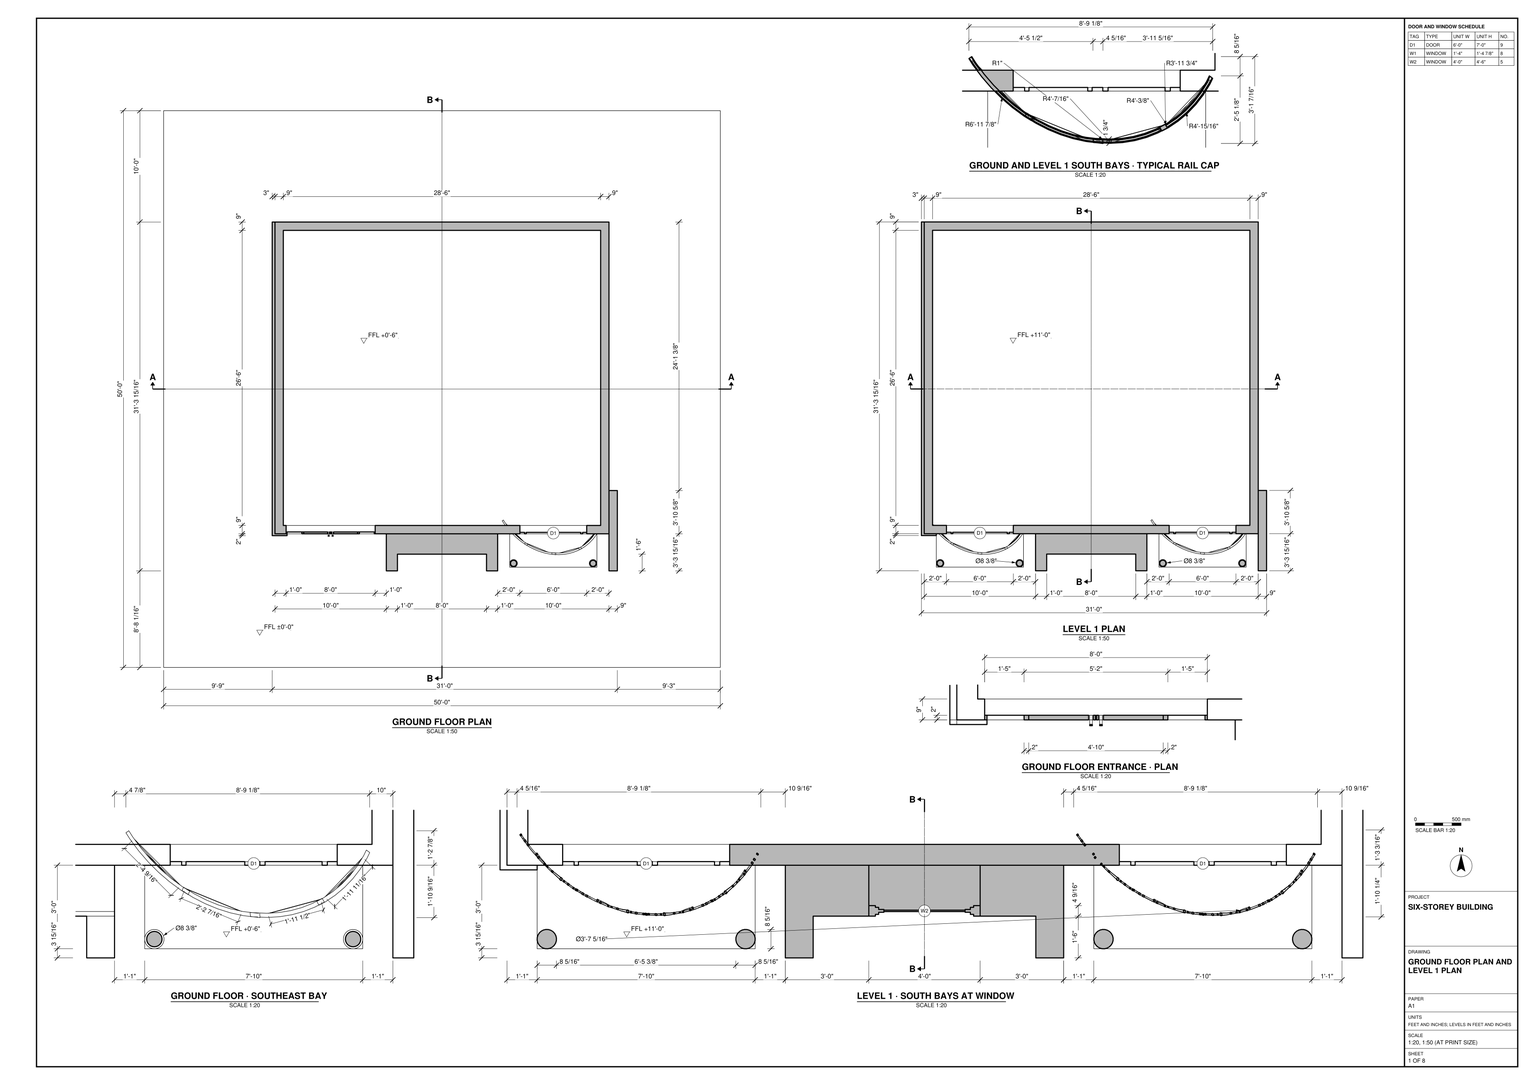
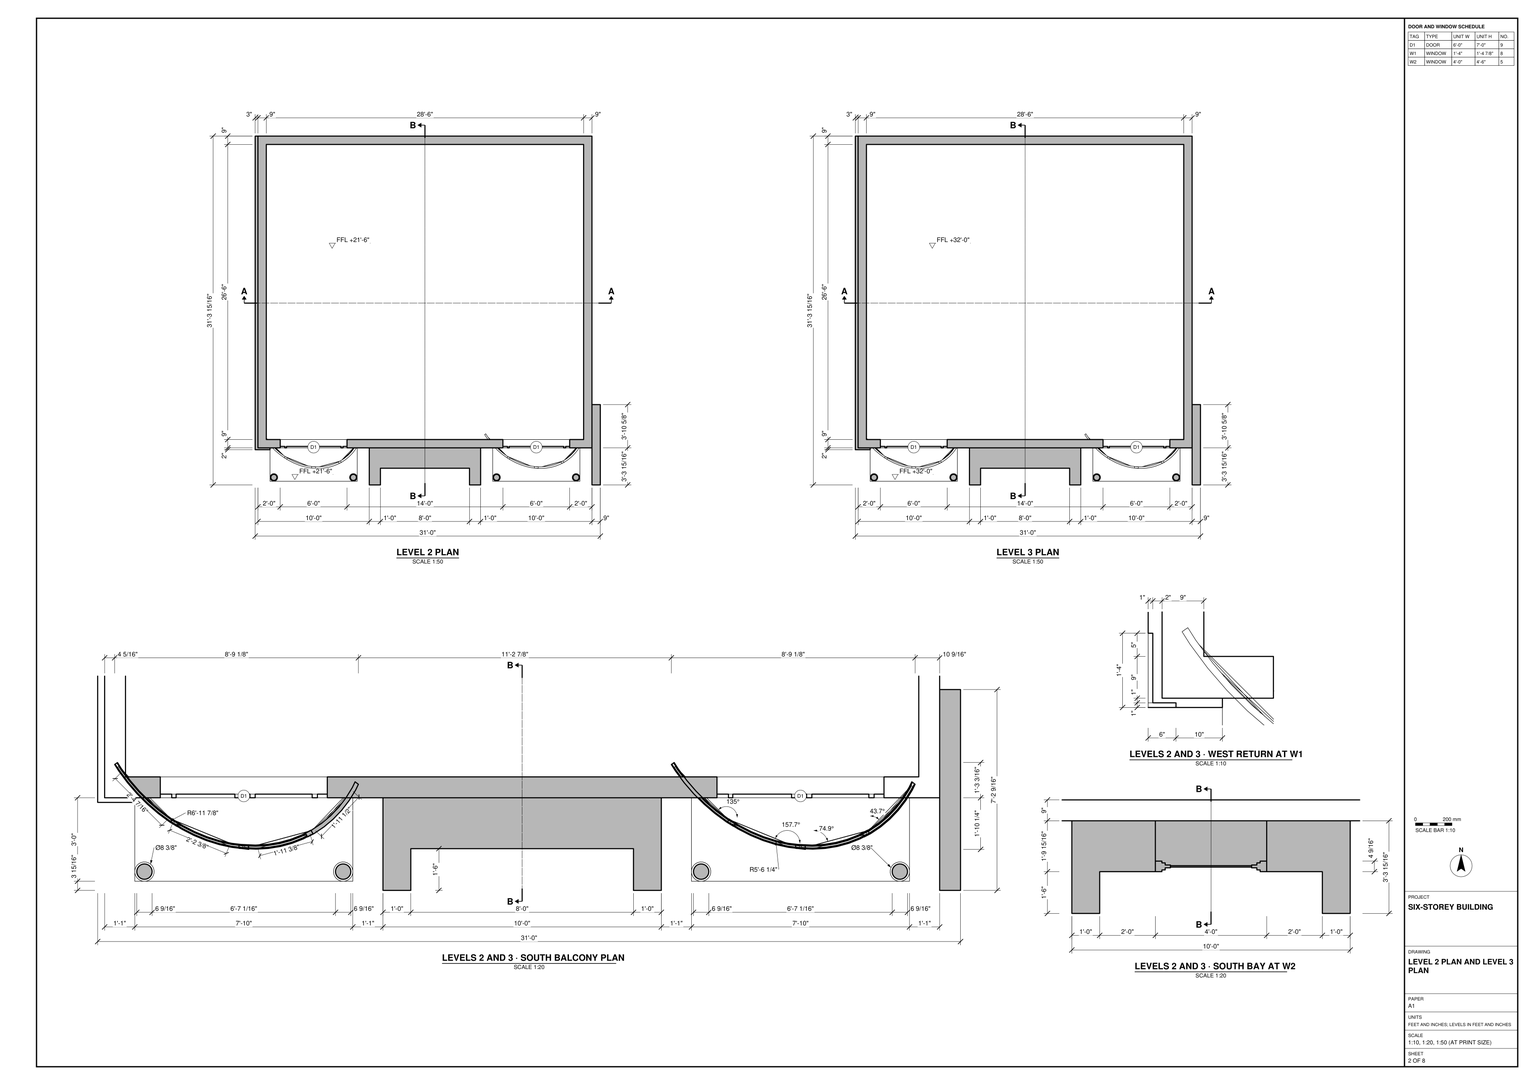
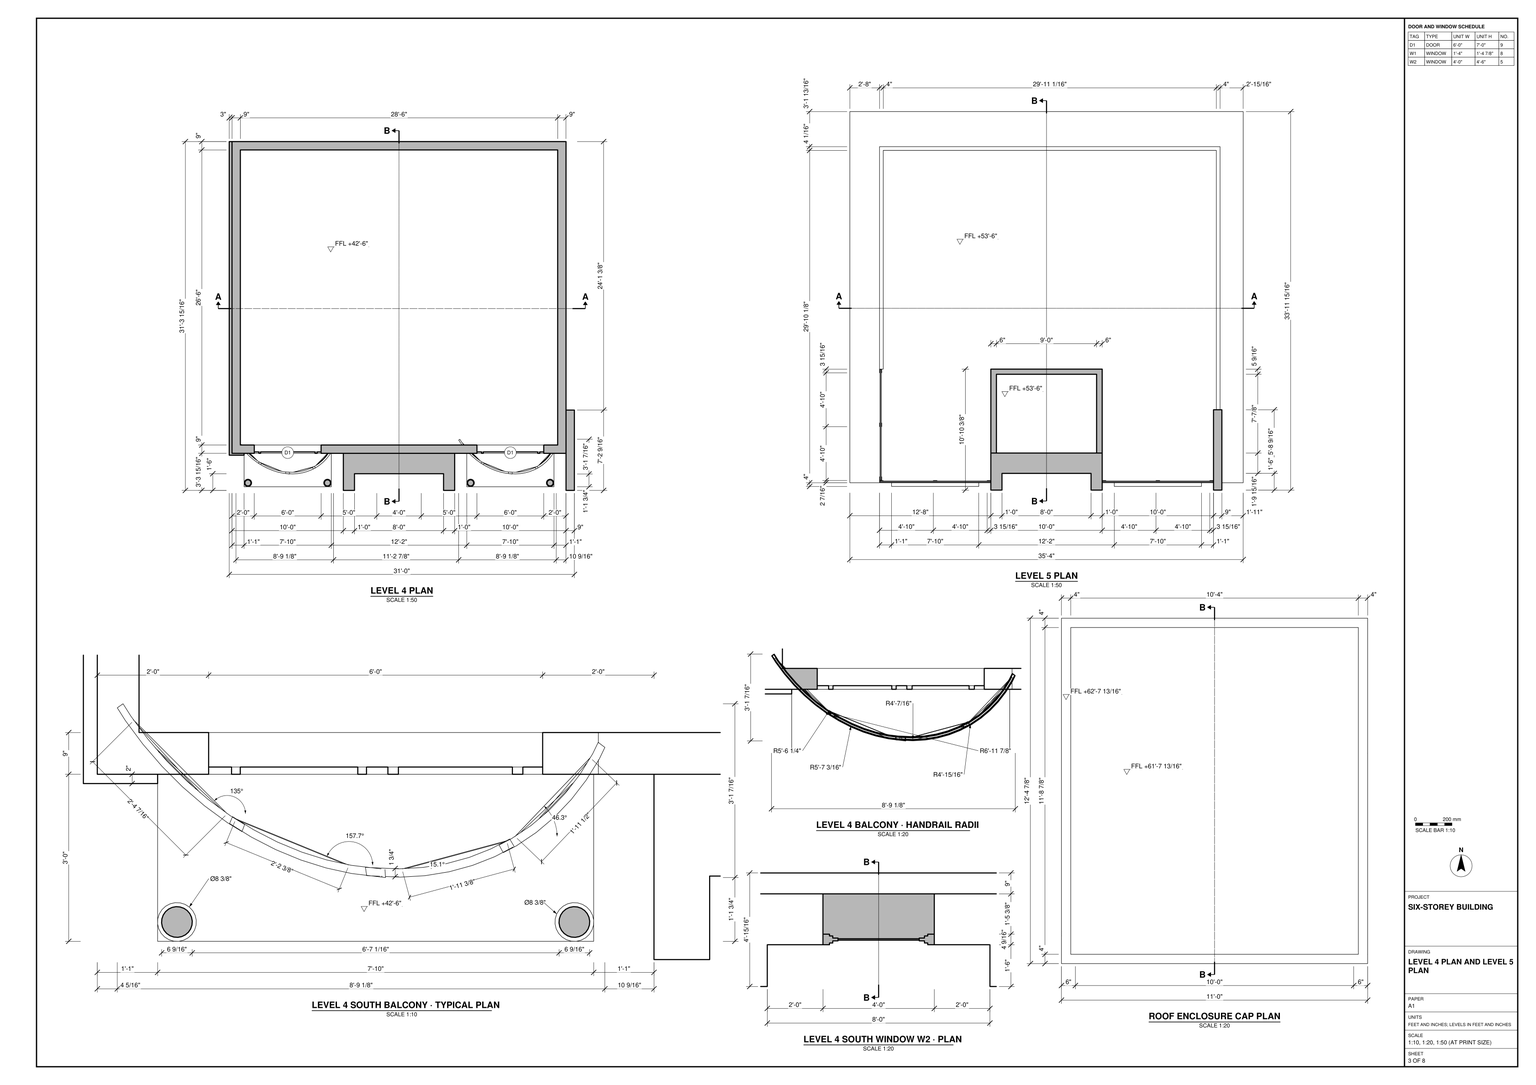
Build the six-storey building in SketchUp from task_files/diagram_01.pdf. Work in feet and inches. Include the square site base: the overall model is 50'-0" wide by 50'-0" deep and 63'-1 13/16" high. Use ±0'-0" as the ground datum and set the upper levels at +11'-0", +21'-6", +32'-0", +42'-6" and +53'-6". Place the ground-floor finished surface at +0'-6", as marked on the plan.

Position the building on the base using the drawn setbacks. Model the floor slabs and perimeter walls, keeping the main floor areas open. Follow the wall thicknesses shown, including the 9" perimeter walls around the typical 28'-6" by 26'-6" clear interior. On the south face, distinguish the ground-floor entrance on the west from the curved rail at the southeast bay. On levels 1 through 4, place the balcony doors on either side of the projecting central window bay. Follow the balcony details for the platforms, round supports and outward curves of the rail caps. At level 5, model the roof terrace and the smaller capped enclosure at its south edge.

Keep walls, slabs and roof elements in separate groups or components, and keep each furniture or joinery piece shown separate as well. Use components for repeated parts. Decor and loose items may use any suitable library components. Save one SketchUp model as output_files/six_storey_building_with_curved_balconies.skp.

# SketchUp Ruby script. Lengths in inches.
U = 1.inch
M = Sketchup.active_model
def pt(a) = Geom::Point3d.new(a.map { |v| v * U })
def face(e, loops, mat)
  f = e.add_face(loops[0].map { |a| pt(a) })
  loops[1..].each { |l| e.add_face(l.map { |a| pt(a) }).erase! }
  f.material = f.back_material = mat if mat
  f
end
# faces: each face lists its corners as indices into pts; further lists are holes
def faces(e, pts, list, mat = nil) = list.each { |f| face(e, (f[0].is_a?(Array) ? f : [f]).map { |l| l.map { |i| pts[i] } }, mat) }
# xy, xz, yz: faces in a plane at the given z, y or x. An outline is a flat list of corners, or four numbers for a rectangle; further outlines are holes
def ring(l) = l.size == 4 ? [[l[0], l[1]], [l[2], l[1]], [l[2], l[3]], [l[0], l[3]]] : l.each_slice(2).to_a
def flat(e, list, mat, &to3) = list.each { |f| face(e, (f[0].is_a?(Array) ? f : [f]).map { |l| ring(l).map { |u, v| to3.(u, v) } }, mat) }
def xy(e, z, list, mat = nil) = flat(e, list, mat) { |x, y| [x, y, z] }
def xz(e, y, list, mat = nil) = flat(e, list, mat) { |x, z| [x, y, z] }
def yz(e, x, list, mat = nil) = flat(e, list, mat) { |y, z| [x, y, z] }
def lines(e, pts, list) = list.each { |a, b| e.add_line(pt(pts[a]), pt(pts[b])) }
# prism: a flat outline (further loops are holes) pulled along v
def prism(e, loops, v, mat = nil)
  f = face(e, loops, mat); d = Geom::Vector3d.new(v.map { |x| x * U })
  f.pushpull(f.normal.samedirection?(d) ? d.length : -d.length)
end
def box(e, o, s, mat = nil) = prism(e, [[o, [o[0] + s[0], o[1], o[2]], [o[0] + s[0], o[1] + s[1], o[2]], [o[0], o[1] + s[1], o[2]]]], [0, 0, s[2]], mat)
def at(x, y, z, deg = 0) = Geom::Transformation.translation(pt([x, y, z])) * Geom::Transformation.rotation(ORIGIN, Z_AXIS, deg.degrees)
def axes(o, x, y, z) = Geom::Transformation.new([*x, 0, *y, 0, *z, 0, *pt(o).to_a, 1])
def part(name) = M.definitions.add(name)
# library, detail: a bought-in or finely detailed component or shape, given as its bounding box
def library(name, o, s) = part(name).tap { |d| box(d.entities, o, s) }
def detail(e, o, s) = box(e.add_group.entities, o, s)
def put(e, d, t, mat = nil) = e.add_instance(d, t).tap { |i| i.material = mat if mat }
def group(e, t, mat = nil) = e.add_group.tap { |g| g.transformation = t; g.material = mat if mat }.entities
root = M.entities
M.materials.add("Egyptian plain").color = [213, 192, 143]
M.materials.add("[0009_Linen]").color = [250, 240, 230]
M.materials.add("[0128_White]").color = [255, 255, 255]
M.materials.add("[0135_DarkGray]").color = [58, 58, 58]
M.materials.add("[Brick_Pavers_Modular]").color = [175, 143, 129]
M.materials.add("[Color_002]").color = [172, 198, 184]
M.materials["[Color_002]"].alpha = 0.07
M.materials.add("[Metal Seamed]").color = [118, 119, 115]
M.materials.add("[Metal Steel Textured White]").color = [191, 191, 191]
M.materials.add("[Stone Flagstone Ashlar]").color = [175, 116, 102]
M.materials.add("[Stone Sandstone Ashlar Light]").color = [206, 178, 128]
M.materials.add("[Suede Dark Gray]").color = [85, 85, 85]
M.materials.add("[Tile Canvas]").color = [199, 192, 173]
M.materials.add("[Translucent Glass Blue]1").color = [36, 54, 86]
M.materials["[Translucent Glass Blue]1"].alpha = 0.5
M.materials.add("[Translucent Glass Gray]").color = [128, 128, 128]
M.materials["[Translucent Glass Gray]"].alpha = 0.5
M.materials.add("[Translucent Glass Sky Reflection]").color = [126, 138, 183]
M.materials["[Translucent Glass Sky Reflection]"].alpha = 0.52
M.materials.add("lotus_tile").color = [249, 184, 163]
c1 = library("Curved balcony railing",[-7.33,0,0],[113.4,71.71,36.05])
c2 = part("french+doors")
xy(c2.entities,5.68,[[49.93,-1.5625,72.3,0]],"[0128_White]")
xy(c2.entities,5.91,[[75.85,-1.5625,98.22,0]],"[0128_White]")
xy(c2.entities,7.12,[[51.37,-1.5625,70.86,0]],"[0128_White]")
xy(c2.entities,7.65,[[77.59,-1.5625,96.49,0]],"[0128_White]")
xy(c2.entities,64.42,[[77.59,-1.5625,96.49,0]],"[0128_White]")
xy(c2.entities,64.48,[[51.37,-1.5625,70.86,0]],"[0128_White]")
xy(c2.entities,65.93,[[49.93,-1.5625,72.3,0]],"[0128_White]")
xy(c2.entities,66.16,[[75.85,-1.5625,98.22,0]],"[0128_White]")
xz(c2.entities,-1.5625,[[[49.93,5.68,72.3,65.93],[51.37,7.12,70.86,64.48]],[[75.85,5.91,98.22,66.16],[77.59,7.65,96.49,64.42]]],"[0128_White]")
xz(c2.entities,0,[[[46.13,3.05,101.5,68.24],[49.93,5.68,72.3,65.93],[75.85,5.91,98.22,66.16]]],"[0128_White]")
xz(c2.entities,0,[[51.37,7.12,70.86,64.48],[77.59,7.65,96.49,64.42]],"[Translucent Glass Gray]")
yz(c2.entities,49.93,[[-1.5625,5.68,0,65.93]],"[0128_White]")
yz(c2.entities,51.37,[[-1.5625,7.12,0,64.48]],"[0128_White]")
yz(c2.entities,70.86,[[-1.5625,7.12,0,64.48]],"[0128_White]")
yz(c2.entities,72.3,[[-1.5625,5.68,0,65.93]],"[0128_White]")
yz(c2.entities,75.85,[[-1.5625,5.91,0,66.16]],"[0128_White]")
yz(c2.entities,77.59,[[-1.5625,7.65,0,64.42]],"[0128_White]")
yz(c2.entities,96.49,[[-1.5625,7.65,0,64.42]],"[0128_White]")
yz(c2.entities,98.22,[[-1.5625,5.91,0,66.16]],"[0128_White]")
c3 = part("Egypt+Pillar")
xy(c3.entities,0,[[[59.76,-0.27,46.92,0.17,34.63,3.93,23.74,10.73,14.97,20.13,8.94,31.47,6.05,43.99,6.5,56.83,10.25,69.11,17.06,80.01,26.45,88.77,37.8,94.8,50.3125,97.7,63.15,97.25,75.4375,93.49,86.33,86.6875,95.1,77.29,101.13,65.95,104.02,53.43,103.57,40.59,99.82,28.31,93.01,17.41,83.62,8.65,72.28,2.62],[57.24,9.8,67.23,11.69,76.4,16.11,84.11,22.75,89.84,31.16,93.19,40.77,93.95,50.91,92.05,60.91,87.64,70.07,81,77.78,72.59,83.51,62.98,86.87,52.83,87.625,42.84,85.73,33.67,81.31,25.96,74.67,20.23,66.26,16.88,56.66,16.12,46.51,18.02,36.51,22.4375,27.35,29.08,19.64,37.49,13.91,47.09,10.55]]])
xy(c3.entities,57.875,[[[59.76,-0.27,72.28,2.62,83.62,8.65,93.01,17.41,99.82,28.31,103.57,40.59,104.02,53.43,101.13,65.95,95.1,77.29,86.33,86.6875,75.4375,93.49,63.15,97.25,50.3125,97.7,37.8,94.8,26.45,88.77,17.06,80.01,10.25,69.11,6.5,56.83,6.05,43.99,8.94,31.47,14.97,20.13,23.74,10.73,34.63,3.93,46.92,0.17],[57.24,9.8,47.09,10.55,37.49,13.91,29.08,19.64,22.4375,27.35,18.02,36.51,16.12,46.51,16.88,56.66,20.23,66.26,25.96,74.67,33.67,81.31,42.84,85.73,52.83,87.625,62.98,86.87,72.59,83.51,81,77.78,87.64,70.07,92.05,60.91,93.95,50.91,93.19,40.77,89.84,31.16,84.11,22.75,76.4,16.11,67.23,11.69]]],"[Brick_Pavers_Modular]")
xy(c3.entities,345.28,[[57.24,9.8,47.09,10.55,37.49,13.91,29.08,19.64,22.4375,27.35,18.02,36.51,16.12,46.51,16.88,56.66,20.23,66.26,25.96,74.67,33.67,81.31,42.84,85.73,52.83,87.625,62.98,86.87,72.59,83.51,81,77.78,87.64,70.07,92.05,60.91,93.95,50.91,93.19,40.77,89.84,31.16,84.11,22.75,76.4,16.11,67.23,11.69]],"[Brick_Pavers_Modular]")
p = [[46.92,0.17,0],[59.76,-0.27,0],[59.76,-0.27,57.875],[46.92,0.17,57.875],[72.28,2.62,0],[72.28,2.62,57.875],
  [34.63,3.93,0],[34.63,3.93,57.875],[83.62,8.65,0],[83.62,8.65,57.875],[23.74,10.73,0],[23.74,10.73,57.875],
  [93.01,17.41,0],[93.01,17.41,57.875],[14.97,20.13,0],[14.97,20.13,57.875],[99.82,28.31,0],[99.82,28.31,57.875],
  [8.94,31.47,0],[8.94,31.47,57.875],[103.57,40.59,0],[103.57,40.59,57.875],[6.05,43.99,0],[6.05,43.99,57.875],
  [104.02,53.43,0],[104.02,53.43,57.875],[6.5,56.83,0],[6.5,56.83,57.875],[101.13,65.95,0],[101.13,65.95,57.875],
  [10.25,69.11,0],[10.25,69.11,57.875],[95.1,77.29,0],[95.1,77.29,57.875],[17.06,80.01,0],[17.06,80.01,57.875],
  [86.33,86.6875,0],[86.33,86.6875,57.875],[26.45,88.77,0],[26.45,88.77,57.875],[75.4375,93.49,0],[75.4375,93.49,57.875],
  [37.8,94.8,0],[37.8,94.8,57.875],[63.15,97.25,0],[63.15,97.25,57.875],[50.3125,97.7,0],[50.3125,97.7,57.875],
  [47.09,10.55,57.875],[57.24,9.8,57.875],[57.24,9.8,345.28],[47.09,10.55,345.28],[67.23,11.69,57.875],[67.23,11.69,345.28],
  [37.49,13.91,57.875],[37.49,13.91,345.28],[76.4,16.11,57.875],[76.4,16.11,345.28],[29.08,19.64,57.875],[29.08,19.64,345.28],
  [84.11,22.75,57.875],[84.11,22.75,345.28],[22.4375,27.35,57.875],[22.4375,27.35,345.28],[89.84,31.16,57.875],[89.84,31.16,345.28],
  [18.02,36.51,57.875],[18.02,36.51,345.28],[93.19,40.77,57.875],[93.19,40.77,345.28],[16.12,46.51,57.875],[16.12,46.51,345.28],
  [93.95,50.91,57.875],[93.95,50.91,345.28],[16.88,56.66,57.875],[16.88,56.66,345.28],[92.05,60.91,57.875],[92.05,60.91,345.28],
  [20.23,66.26,57.875],[20.23,66.26,345.28],[87.64,70.07,57.875],[87.64,70.07,345.28],[25.96,74.67,57.875],[25.96,74.67,345.28],
  [81,77.78,57.875],[81,77.78,345.28],[33.67,81.31,57.875],[33.67,81.31,345.28],[72.59,83.51,57.875],[72.59,83.51,345.28],
  [42.84,85.73,57.875],[42.84,85.73,345.28],[62.98,86.87,57.875],[62.98,86.87,345.28],[52.83,87.625,57.875],[52.83,87.625,345.28],
  [52.83,87.625,0],[62.98,86.87,0],[42.84,85.73,0],[33.67,81.31,0],[25.96,74.67,0],[20.23,66.26,0],
  [16.88,56.66,0],[16.12,46.51,0],[18.02,36.51,0],[22.4375,27.35,0],[29.08,19.64,0],[37.49,13.91,0],
  [47.09,10.55,0],[57.24,9.8,0],[67.23,11.69,0],[76.4,16.11,0],[84.11,22.75,0],[89.84,31.16,0],
  [93.19,40.77,0],[93.95,50.91,0],[92.05,60.91,0],[87.64,70.07,0],[81,77.78,0],[72.59,83.51,0]]
faces(c3.entities,p,[[0,1,2,3],[1,4,5,2],[6,0,3,7],[4,8,9,5],[10,6,7,11],[8,12,13,9],[14,10,11,15],[12,16,17,13],
  [18,14,15,19],[16,20,21,17],[22,18,19,23],[20,24,25,21],[26,22,23,27],[24,28,29,25],[30,26,27,31],[28,32,33,29],
  [34,30,31,35],[32,36,37,33],[38,34,35,39],[36,40,41,37],[42,38,39,43],[40,44,45,41],[46,42,43,47],[44,46,47,45]],"lotus_tile")
faces(c3.entities,p,[[48,49,50,51],[49,52,53,50],[54,48,51,55],[52,56,57,53],[58,54,55,59],[56,60,61,57],[62,58,59,63],[60,64,65,61],
  [66,62,63,67],[64,68,69,65],[70,66,67,71],[68,72,73,69],[74,70,71,75],[72,76,77,73],[78,74,75,79],[76,80,81,77],
  [82,78,79,83],[80,84,85,81],[86,82,83,87],[84,88,89,85],[90,86,87,91],[88,92,93,89],[94,90,91,95],[92,94,95,93]],"Egyptian plain")
lines(c3.entities,p,[[96,94],[97,92],[98,90],[99,86],[100,82],[101,78],[102,74],[103,70],[104,66],[105,62],[106,58],[107,54],
  [108,48],[109,49],[110,52],[111,56],[112,60],[113,64],[114,68],[115,72],[116,76],[117,80],[118,84],[119,88]])
c4 = part("Mounting plate")
xy(c4.entities,-0.08,[[2.57,0.63,2.46,0.64,2.36,0.69,2.28,0.75,2.21,0.84,2.17,0.9375,2.15,1.05,2.17,1.15,2.21,1.25,2.27,1.34,2.36,1.41,2.46,1.45,2.57,1.46,2.68,1.45,2.78,1.41,2.86,1.34,2.93,1.26,2.97,1.16,2.99,1.05,2.97,0.94,2.93,0.84,2.87,0.75,2.78,0.6875,2.68,0.64]])
xy(c4.entities,0,[[0.79,0,0.68,0.01,0.58,0.03,0.49,0.06,0.39,0.11,0.31,0.16,0.23,0.23,0.16,0.31,0.11,0.39,0.06,0.49,0.03,0.58,0.01,0.68,0,0.79,0,1.1,0.01,1.21,0.03,1.31,0.06,1.4,0.11,1.5,0.16,1.58,0.23,1.66,0.31,1.73,0.39,1.78,0.49,1.83,0.58,1.86,0.68,1.88,0.79,1.89,7.875,1.89,7.875,0]])
xy(c4.entities,0.2,[[[0.79,0,0.68,0.01,0.58,0.03,0.49,0.06,0.39,0.11,0.31,0.16,0.23,0.23,0.16,0.31,0.11,0.39,0.06,0.49,0.03,0.58,0.01,0.68,0,0.79,0,1.1,0.01,1.21,0.03,1.31,0.06,1.4,0.11,1.5,0.16,1.58,0.23,1.66,0.31,1.73,0.39,1.78,0.49,1.83,0.58,1.86,0.68,1.88,0.79,1.89,7.875,1.89,7.875,0],[2.57,0.63,2.68,0.64,2.78,0.6875,2.87,0.75,2.93,0.84,2.97,0.94,2.99,1.05,2.97,1.16,2.93,1.26,2.86,1.34,2.78,1.41,2.68,1.45,2.57,1.46,2.46,1.45,2.36,1.41,2.27,1.34,2.21,1.25,2.17,1.15,2.15,1.05,2.17,0.9375,2.21,0.84,2.28,0.75,2.36,0.69,2.46,0.64]],[2.57,0.63,2.68,0.64,2.78,0.6875,2.87,0.75,2.93,0.84,2.97,0.94,2.99,1.05,2.97,1.16,2.93,1.26,2.86,1.34,2.78,1.41,2.68,1.45,2.57,1.46,2.46,1.45,2.36,1.41,2.27,1.34,2.21,1.25,2.17,1.15,2.15,1.05,2.17,0.9375,2.21,0.84,2.28,0.75,2.36,0.69,2.46,0.64]])
xy(c4.entities,0.68,[[2.57,0.63,2.46,0.64,2.36,0.69,2.28,0.75,2.21,0.84,2.17,0.9375,2.15,1.05,2.17,1.15,2.21,1.25,2.27,1.34,2.36,1.41,2.46,1.45,2.57,1.46,2.68,1.45,2.78,1.41,2.86,1.34,2.93,1.26,2.97,1.16,2.99,1.05,2.97,0.94,2.93,0.84,2.87,0.75,2.78,0.6875,2.68,0.64]])
xz(c4.entities,0,[[0.79,0,7.875,0.2]])
xz(c4.entities,1.89,[[0.79,0,7.875,0.08],[0.79,0.08,7.875,0.2]])
yz(c4.entities,0,[[0.79,0,1.1,0.08],[0.79,0.08,1.1,0.2]])
p = [[2.46,0.64,-0.08],[2.46,0.64,0.2],[2.36,0.69,0.2],[2.36,0.69,-0.08],[2.57,0.63,-0.08],[2.57,0.63,0.2],
  [2.68,0.64,-0.08],[2.68,0.64,0.2],[2.78,0.6875,-0.08],[2.78,0.6875,0.2],[2.28,0.75,0.2],[2.28,0.75,-0.08],
  [2.87,0.75,-0.08],[2.87,0.75,0.2],[2.21,0.84,-0.08],[2.21,0.84,0.2],[2.17,0.9375,0.2],[2.17,0.9375,-0.08],
  [2.93,0.84,-0.08],[2.93,0.84,0.2],[2.97,0.94,-0.08],[2.97,0.94,0.2],[2.15,1.05,0.2],[2.15,1.05,-0.08],
  [2.99,1.05,-0.08],[2.99,1.05,0.2],[2.17,1.15,0.2],[2.17,1.15,-0.08],[2.97,1.16,-0.08],[2.97,1.16,0.2],
  [2.21,1.25,0.2],[2.21,1.25,-0.08],[2.93,1.26,-0.08],[2.93,1.26,0.2],[2.27,1.34,0.2],[2.27,1.34,-0.08],
  [2.36,1.41,0.2],[2.36,1.41,-0.08],[2.78,1.41,-0.08],[2.78,1.41,0.2],[2.86,1.34,0.2],[2.86,1.34,-0.08],
  [2.46,1.45,0.2],[2.46,1.45,-0.08],[2.68,1.45,-0.08],[2.68,1.45,0.2],[2.57,1.46,0.2],[2.57,1.46,-0.08],
  [0.49,0.06,0.2],[0.49,0.06,0],[0.58,0.03,0],[0.58,0.03,0.2],[0.68,0.01,0],[0.68,0.01,0.2],
  [0.79,0,0],[0.79,0,0.2],[0.31,0.16,0.2],[0.31,0.16,0.08],[0.31,0.16,0],[0.39,0.11,0],
  [0.39,0.11,0.2],[0.23,0.23,0],[0.23,0.23,0.08],[0.16,0.31,0.08],[0.16,0.31,0],[0.11,0.39,0.08],
  [0.11,0.39,0],[0.06,0.49,0.08],[0.06,0.49,0],[0.03,0.58,0.08],[0.03,0.58,0],[0.01,0.68,0.08],
  [0.01,0.68,0],[0,0.79,0.08],[0,0.79,0],[0,1.1,0],[0,1.1,0.08],[0.01,1.21,0.08],
  [0.01,1.21,0],[0.03,1.31,0.08],[0.03,1.31,0],[0.06,1.4,0.08],[0.06,1.4,0],[0.11,1.5,0.08],
  [0.11,1.5,0],[0.16,1.58,0.08],[0.16,1.58,0],[0.23,1.66,0.08],[0.23,1.66,0],[0.31,1.73,0.08],
  [0.31,1.73,0],[0.39,1.78,0.08],[0.39,1.78,0],[0.49,1.83,0.08],[0.49,1.83,0],[0.58,1.86,0.08],
  [0.58,1.86,0],[0.68,1.88,0.08],[0.68,1.88,0],[0.79,1.89,0.08],[0.79,1.89,0],[0.23,0.23,0.2],
  [0.16,0.31,0.2],[0.11,0.39,0.2],[0.06,0.49,0.2],[0.03,0.58,0.2],[0.01,0.68,0.2],[0,0.79,0.2],
  [0,1.1,0.2],[0.01,1.21,0.2],[0.03,1.31,0.2],[0.06,1.4,0.2],[0.11,1.5,0.2],[0.16,1.58,0.2],
  [0.23,1.66,0.2],[0.31,1.73,0.2],[0.39,1.78,0.2],[0.49,1.83,0.2],[0.58,1.86,0.2],[0.68,1.88,0.2],
  [0.79,1.89,0.2],[2.46,0.64,0.68],[2.36,0.69,0.68],[2.57,0.63,0.68],[2.68,0.64,0.68],[2.78,0.6875,0.68],
  [2.28,0.75,0.68],[2.87,0.75,0.68],[2.21,0.84,0.68],[2.17,0.9375,0.68],[2.97,0.94,0.68],[2.93,0.84,0.68],
  [2.15,1.05,0.68],[2.99,1.05,0.68],[2.17,1.15,0.68],[2.97,1.16,0.68],[2.21,1.25,0.68],[2.93,1.26,0.68],
  [2.27,1.34,0.68],[2.36,1.41,0.68],[2.78,1.41,0.68],[2.86,1.34,0.68],[2.46,1.45,0.68],[2.68,1.45,0.68],
  [2.57,1.46,0.68]]
faces(c4.entities,p,[[0,1,2,3],[4,5,1,0],[6,7,5,4],[8,9,7,6],[3,2,10,11],[12,13,9,8],[14,15,16,17],[11,10,15,14],
  [18,19,13,12],[20,21,19,18],[17,16,22,23],[24,25,21,20],[23,22,26,27],[28,29,25,24],[27,26,30,31],[32,33,29,28],
  [31,30,34,35],[35,34,36,37],[38,39,40,41],[41,40,33,32],[37,36,42,43],[44,45,39,38],[43,42,46,47],[47,46,45,44],
  [48,49,50,51],[51,50,52,53],[53,52,54,55],[56,57,58,59,60],[60,59,49,48],[61,62,63,64],[58,57,62,61],[64,63,65,66],
  [66,65,67,68],[68,67,69,70],[70,69,71,72],[72,71,73,74],[75,76,77,78],[78,77,79,80],[80,79,81,82],[82,81,83,84],
  [84,83,85,86],[86,85,87,88],[88,87,89,90],[90,89,91,92],[92,91,93,94],[94,93,95,96],[96,95,97,98],[98,97,99,100],
  [63,62,101,102],[62,57,56,101],[65,63,102,103],[67,65,103,104],[69,67,104,105],[71,69,105,106],[73,71,106,107],[77,76,108,109],
  [79,77,109,110],[81,79,110,111],[83,81,111,112],[85,83,112,113],[87,85,113,114],[89,87,114,115],[91,89,115,116],[93,91,116,117],
  [95,93,117,118],[97,95,118,119],[99,97,119,120],[2,1,121,122],[1,5,123,121],[5,7,124,123],[7,9,125,124],[10,2,122,126],
  [9,13,127,125],[15,10,126,128],[16,15,128,129],[19,21,130,131],[13,19,131,127],[22,16,129,132],[21,25,133,130],[26,22,132,134],
  [25,29,135,133],[30,26,134,136],[29,33,137,135],[34,30,136,138],[36,34,138,139],[40,39,140,141],[33,40,141,137],[42,36,139,142],
  [39,45,143,140],[46,42,142,144],[45,46,144,143]])
c5 = part("Glass panel railing")
xy(c5.entities,0,[[0,0,3.9375,6.3],[0,92.32,3.9375,98.62],[0,184.64,3.9375,190.9375]],"[Metal Seamed]")
xy(c5.entities,0.39,[[0,0,3.9375,1.57],[0,1.57,1.18,4.72],[1.18,1.57,1.97,4.72],[1.97,1.57,2.76,4.72],[2.76,1.57,3.9375,4.72],
  [0,4.72,3.9375,6.3],[0,92.32,3.9375,93.89],[0,93.89,1.18,97.04],[1.18,93.89,1.97,97.04],[1.97,93.89,2.76,97.04],
  [2.76,93.89,3.9375,97.04],[0,97.04,3.9375,98.62],[0,184.64,3.9375,186.21],[0,186.21,1.18,189.36],[1.18,186.21,1.97,189.36],
  [1.97,186.21,2.76,189.36],[2.76,186.21,3.9375,189.36],[0,189.36,3.9375,190.9375]],"[Metal Seamed]")
xy(c5.entities,5.55,[[1.46,7.875,1.85,90.76]],"[Color_002]")
xy(c5.entities,60.67,[[1.46,7.875,1.85,90.76]],"[Color_002]")
xy(c5.entities,62.2,[[[0.79,0.57,1.18,0.57,1.18,4.72,2.76,4.72,2.76,0.57,3.15,0.57,3.15,190.36,2.76,190.36,2.76,186.21,1.18,186.21,1.18,190.36,0.79,190.36],[1.18,93.89,2.76,97.04]],[1.18,0.57,1.97,1.57],[1.97,0.57,2.76,1.57],[1.18,1.57,1.97,2.36],[1.97,1.57,2.76,2.36],
  [1.18,2.36,1.57,3.9375],[1.57,2.36,1.97,3.9375],[1.97,2.36,2.36,3.9375],[2.36,2.36,2.76,3.9375],[1.18,3.9375,1.97,4.72],
  [1.97,3.9375,2.76,4.72],[1.18,93.89,1.97,94.68],[1.97,93.89,2.76,94.68],[1.18,94.68,1.57,96.26],[1.57,94.68,1.97,96.26],
  [1.97,94.68,2.36,96.26],[2.36,94.68,2.76,96.26],[1.18,96.26,1.97,97.04],[1.97,96.26,2.76,97.04],[1.18,186.21,1.97,187],
  [1.97,186.21,2.76,187],[1.18,187,1.57,188.58],[1.57,187,1.97,188.58],[1.97,187,2.36,188.58],[2.36,187,2.76,188.58],
  [1.18,188.58,1.97,189.36],[1.97,188.58,2.76,189.36],[1.18,189.36,1.97,190.36],[1.97,189.36,2.76,190.36]],"[Metal Seamed]")
xy(c5.entities,64.57,[[0.79,0.57,1.97,190.36],[1.97,0.57,3.15,190.36]],"[Metal Seamed]")
xz(c5.entities,0,[[0,0,3.9375,0.39]],"[Metal Seamed]")
xz(c5.entities,0.57,[[0.79,62.2,3.15,64.57]],"[Metal Seamed]")
xz(c5.entities,1.57,[[1.18,0.39,2.76,62.2]],"[Metal Seamed]")
xz(c5.entities,4.72,[[1.18,0.39,2.76,13.9375],[1.18,13.9375,2.76,50.39],[1.18,50.39,2.76,62.2]],"[Metal Seamed]")
xz(c5.entities,6.3,[[0,0,3.9375,0.39]],"[Metal Seamed]")
xz(c5.entities,7.875,[[1.46,5.55,1.85,60.67]],"[Color_002]")
xz(c5.entities,90.76,[[1.46,5.55,1.85,60.67]],"[Color_002]")
xz(c5.entities,92.32,[[0,0,3.9375,0.39]],"[Metal Seamed]")
xz(c5.entities,93.89,[[1.18,0.39,2.76,62.2]],"[Metal Seamed]")
xz(c5.entities,97.04,[[1.18,0.39,2.76,13.9375],[1.18,13.9375,2.76,50.39],[1.18,50.39,2.76,62.2]],"[Metal Seamed]")
xz(c5.entities,98.62,[[0,0,3.9375,0.39]],"[Metal Seamed]")
xz(c5.entities,184.64,[[0,0,3.9375,0.39]],"[Metal Seamed]")
xz(c5.entities,186.21,[[1.18,0.39,2.76,62.2]],"[Metal Seamed]")
xz(c5.entities,189.36,[[1.18,0.39,2.76,13.9375],[1.18,13.9375,2.76,50.39],[1.18,50.39,2.76,62.2]],"[Metal Seamed]")
xz(c5.entities,190.36,[[0.79,62.2,3.15,64.57]],"[Metal Seamed]")
xz(c5.entities,190.9375,[[0,0,3.9375,0.39]],"[Metal Seamed]")
yz(c5.entities,0,[[0,0,6.3,0.39],[92.32,0,98.62,0.39],[184.64,0,190.9375,0.39]],"[Metal Seamed]")
yz(c5.entities,0.79,[[0.57,62.2,190.36,64.57]],"[Metal Seamed]")
yz(c5.entities,1.18,[[1.57,0.39,4.72,62.2],[93.89,0.39,97.04,62.2],[186.21,0.39,189.36,62.2]],"[Metal Seamed]")
yz(c5.entities,1.46,[[7.875,5.55,90.76,60.67]],"[Color_002]")
yz(c5.entities,1.85,[[7.875,5.55,90.76,60.67],[100.19,5.55,183.08,60.67]],"[Translucent Glass Gray]")
yz(c5.entities,2.76,[[1.57,0.39,4.72,62.2],[93.89,0.39,97.04,62.2],[186.21,0.39,189.36,62.2]],"[Metal Seamed]")
yz(c5.entities,3.15,[[0.57,62.2,190.36,64.57]],"[Metal Seamed]")
yz(c5.entities,3.9375,[[0,0,6.3,0.39],[92.32,0,98.62,0.39],[184.64,0,190.9375,0.39]],"[Metal Seamed]")
p = [[1.85,100.19,7.77],[1.85,100.18,7.91],[1.46,183.08,5.55],[1.85,183.08,5.55],[1.85,183.08,60.67],[1.46,183.08,60.67],
  [1.46,100.19,5.55],[1.85,100.19,5.55],[1.46,100.21,7.61],[1.46,100.19,7.77],[1.46,100.19,60.67],[1.85,100.19,60.67],
  [1.85,7.875,58.45],[1.85,7.86,58.31]]
lines(c5.entities,p,[[0,1],[2,3],[4,5],[6,7],[8,9],[10,9],[11,10],[12,13],[6,8]])
put(c5.entities,c4,axes([2.05,86.02,12.05],[0,1,0],[0,0,1],[-1,0,0]),"[Metal Steel Textured White]")
put(c5.entities,c4,axes([2.05,12.6,48.5],[0,-1,0],[0,0,1],[-1,0,0]),"[Metal Steel Textured White]")
put(c5.entities,c4,axes([2.05,12.6,12.05],[0,-1,0],[0,0,1],[-1,0,0]),"[Metal Steel Textured White]")
put(c5.entities,c4,axes([2.05,178.34,48.5],[0,1,0],[0,0,1],[-1,0,0]),"[Metal Steel Textured White]")
put(c5.entities,c4,axes([2.05,86.02,48.5],[0,1,0],[0,0,1],[-1,0,0]),"[Metal Steel Textured White]")
put(c5.entities,c4,axes([2.05,104.92,12.05],[0,-1,0],[0,0,1],[-1,0,0]),"[Metal Steel Textured White]")
put(c5.entities,c4,axes([2.05,104.92,48.5],[0,-1,0],[0,0,1],[-1,0,0]),"[Metal Steel Textured White]")
put(c5.entities,c4,axes([2.05,178.34,12.05],[0,1,0],[0,0,1],[-1,0,0]),"[Metal Steel Textured White]")
c6 = library("Group\#4",[0,0,0],[96,4.5,84])
c7 = part("Group\#2")
xy(c7.entities,0,[[0,0,360,336]])
xy(c7.entities,6,[[0,0,0,336,360,336,360,0,336,0,336,9,351,9,351,327,9,327,9,9,24,9,24,0],[24,0,96,9],[96,0,108,9],[108,0,264,9],[264,0,336,9],
  [9,9,351,327]])
xy(c7.entities,90,[[24,0,96,9],[264,0,336,9]])
xy(c7.entities,126,[[[0,0,360,336],[9,9,351,327]]])
xz(c7.entities,0,[[0,0,360,6],[0,6,24,6,24,90,96,90,96,6,120,6,120,126,0,126],[120,6,240,126],[240,6,264,6,264,90,336,90,336,6,360,6,360,126,240,126]])
xz(c7.entities,9,[[9,6,9,126,351,126,351,6,336,6,336,90,264,90,264,6,96,6,96,90,24,90,24,6]])
xz(c7.entities,327,[[9,6,351,126]])
xz(c7.entities,336,[[0,0,360,6],[0,6,360,126]])
yz(c7.entities,0,[[0,0,336,6],[0,6,336,126]])
yz(c7.entities,9,[[9,6,327,126]])
yz(c7.entities,24,[[0,6,9,90]])
yz(c7.entities,96,[[0,6,9,90]])
yz(c7.entities,264,[[0,6,9,90]])
yz(c7.entities,336,[[0,6,9,90]])
yz(c7.entities,351,[[9,6,327,126]])
yz(c7.entities,360,[[0,0,336,6],[0,6,336,126]])
c8 = library("Group\#20",[-6.18,-12.5,0],[115.62,108.625,126])
c9 = library("Group\#23",[-6.18,-12.5,0],[115.62,108.625,126])
c10 = library("Group\#17",[-6.18,-12.5,0],[115.62,108.625,126])
c11 = library("Group\#7",[-6.18,-12.5,0],[115.62,108.625,126])
c12 = library("Group\#35",[-6.18,-12.5,0],[115.62,108.625,126])
c13 = library("Group\#37",[-6.18,-12.5,0],[115.62,108.625,126])
c14 = library("Group\#25",[-6.18,-12.5,0],[115.62,108.625,126])
c15 = library("Group\#33",[-6.18,-12.5,0],[115.62,108.625,126])
c16 = part("Glass+Window")
g1 = group(c16.entities,at(0,0,0))
xy(g1,0,[[0,0,5.91,33.46]],"[0135_DarkGray]")
xy(g1,1.97,[[0,1.97,0.98,31.5],[4.92,1.97,5.91,31.5]],"[0135_DarkGray]")
xy(g1,2.95,[[0.98,2.95,2.17,30.51],[3.74,2.95,4.92,30.51]],"[0135_DarkGray]")
xy(g1,4.53,[[2.17,4.53,2.56,28.9375],[2.56,4.53,3.35,28.9375],[3.35,4.53,3.74,28.9375]],"[0135_DarkGray]")
xy(g1,38.78,[[2.17,4.53,2.56,28.9375],[2.56,4.53,3.35,28.9375],[3.35,4.53,3.74,28.9375]],"[0135_DarkGray]")
xy(g1,40.35,[[0.98,2.95,2.17,30.51],[3.74,2.95,4.92,30.51]],"[0135_DarkGray]")
xy(g1,41.34,[[0,1.97,0.98,31.5],[4.92,1.97,5.91,31.5]],"[0135_DarkGray]")
xy(g1,43.31,[[0,0,5.91,33.46]],"[0135_DarkGray]")
xz(g1,0,[[0,0,5.91,43.31]],"[0135_DarkGray]")
xz(g1,1.97,[[0,1.97,0.98,41.34],[4.92,1.97,5.91,41.34]],"[0135_DarkGray]")
xz(g1,2.95,[[0.98,2.95,2.17,40.35],[3.74,2.95,4.92,40.35]],"[0135_DarkGray]")
xz(g1,4.53,[[2.17,4.53,2.56,38.78],[2.56,4.53,3.35,38.78],[3.35,4.53,3.74,38.78]],"[0135_DarkGray]")
xz(g1,28.9375,[[2.17,4.53,2.56,38.78],[2.56,4.53,3.35,38.78],[3.35,4.53,3.74,38.78]],"[0135_DarkGray]")
xz(g1,30.51,[[0.98,2.95,2.17,40.35],[3.74,2.95,4.92,40.35]],"[0135_DarkGray]")
xz(g1,31.5,[[0,1.97,0.98,41.34],[4.92,1.97,5.91,41.34]],"[0135_DarkGray]")
xz(g1,33.46,[[0,0,5.91,43.31]],"[0135_DarkGray]")
yz(g1,0,[[[0,0,33.46,43.31],[1.97,1.97,31.5,41.34]]],"[0135_DarkGray]")
yz(g1,0.98,[[[1.97,1.97,31.5,41.34],[2.95,2.95,30.51,40.35]]],"[0135_DarkGray]")
yz(g1,2.17,[[[2.95,2.95,30.51,40.35],[4.53,4.53,28.9375,38.78]],[30.51,2.95,31.5,4.53]],"[0135_DarkGray]")
yz(g1,2.56,[[4.53,4.53,28.9375,38.78]],"[Translucent Glass Sky Reflection]")
yz(g1,3.35,[[4.53,4.53,28.9375,38.78]],"[Translucent Glass Blue]1")
yz(g1,3.74,[[[2.95,2.95,30.51,40.35],[4.53,4.53,28.9375,38.78]],[30.51,2.95,31.5,4.53]],"[0135_DarkGray]")
yz(g1,4.92,[[[1.97,1.97,31.5,41.34],[2.95,2.95,30.51,40.35]]],"[0135_DarkGray]")
yz(g1,5.91,[[[0,0,33.46,43.31],[1.97,1.97,31.5,41.34]]],"[0135_DarkGray]")
c17 = part("Group\#28")
xy(c17.entities,-16,[[0,1.41,1,2.8125],[0,4.22,1,5.625],[0,7.03,1,8.4375],[0,9.84,1,11.25],[0,12.66,1,14.0625],
  [0,15.47,1,16.875]])
xy(c17.entities,-1,[[1,1.41,6,2.8125],[1,4.22,6,5.625],[1,7.03,6,8.4375],[1,9.84,6,11.25],[1,12.66,6,14.0625],
  [1,15.47,6,16.875]])
xy(c17.entities,0,[[0,0,6,1.41],[0,2.8125,6,4.22],[0,5.625,6,7.03],[0,8.4375,6,9.84],[0,11.25,6,12.66],
  [0,14.0625,6,15.47]])
xz(c17.entities,1.41,[[0,-16,1,-1],[0,-1,6,0]])
xz(c17.entities,2.8125,[[0,-16,1,-1],[0,-1,6,0]])
xz(c17.entities,4.22,[[0,-16,1,-1],[0,-1,6,0]])
xz(c17.entities,5.625,[[0,-16,1,-1],[0,-1,6,0]])
xz(c17.entities,7.03,[[0,-16,1,-1],[0,-1,6,0]])
xz(c17.entities,8.4375,[[0,-16,1,-1],[0,-1,6,0]])
xz(c17.entities,9.84,[[0,-16,1,-1],[0,-1,6,0]])
xz(c17.entities,11.25,[[0,-16,1,-1],[0,-1,6,0]])
xz(c17.entities,12.66,[[0,-16,1,-1],[0,-1,6,0]])
xz(c17.entities,14.0625,[[0,-16,1,-1],[0,-1,6,0]])
xz(c17.entities,15.47,[[0,-16,1,-1],[0,-1,6,0]])
xz(c17.entities,16.875,[[0,-16,1,-1],[0,-1,6,0]])
yz(c17.entities,0,[[0,-16,1.41,0],[2.8125,-16,4.22,0],[5.625,-16,7.03,0],[8.4375,-16,9.84,0],[11.25,-16,12.66,0],
  [14.0625,-16,15.47,0]])
yz(c17.entities,1,[[1.41,-16,2.8125,-1],[4.22,-16,5.625,-1],[7.03,-16,8.4375,-1],[9.84,-16,11.25,-1],[12.66,-16,14.0625,-1],
  [15.47,-16,16.875,-1]])
yz(c17.entities,6,[[1.41,-1,2.8125,0],[4.22,-1,5.625,0],[7.03,-1,8.4375,0],[9.84,-1,11.25,0],[12.66,-1,14.0625,0],
  [15.47,-1,16.875,0]])
p = [[0,16.875,0],[0,0,0]]
lines(c17.entities,p,[[0,1]])
put(root,c1,axes([400.55,98.22,11.95],[0.69576,0.41475,0],[-0.51204,0.85896,0],[0,0,1]))
put(root,c2,axes([324.02,145.5625,8.07],[1.30023,0,0],[0,1,0],[0,0,1.28859]))
put(root,c3,axes([458.16,108.02,12],[0.085,0,0],[0,0.085,0],[0,0,0.24328]))
put(root,c3,axes([372.49,108.02,12],[0.085,0,0],[0,0.085,0],[0,0,0.24328]))
put(root,c5,axes([360,114.44,648],[0,-0.62,0],[0.62848,0,0],[0,0,0.55698]))
put(root,c5,axes([120,114.44,648],[0,-0.62,0],[0.62848,0,0],[0,0,0.55698]))
put(root,c5,axes([120,114.44,648],[0.62,0,0],[0,0.62848,0],[0,0,0.55698]))
g2 = group(root,at(0,0,0))
box(g2,[0,0,0],[600,600,6])
g3 = group(root,at(120,144,6),"[0009_Linen]")
xy(g3,0,[[0,0,360,336]])
xy(g3,6,[[0,0,0,336,360,336,360,0,336,0,336,9,351,9,351,327,9,327,9,9,12,9,12,0],[12,0,108,9],[108,0,264,9],[264,0,336,9],[9,9,351,327]])
xy(g3,90,[[12,0,108,9],[264,0,336,9]])
xy(g3,126,[[[0,0,360,336],[9,9,351,327]]])
xz(g3,0,[[0,0,360,6],[0,6,12,6,12,90,108,90,108,6,120,6,120,126,0,126],[120,6,240,126],[240,6,264,6,264,90,336,90,336,6,360,6,360,126,240,126]])
xz(g3,9,[[9,6,9,126,351,126,351,6,336,6,336,90,264,90,264,6,108,6,108,90,12,90,12,6]])
xz(g3,327,[[9,6,351,126]])
xz(g3,336,[[0,0,360,6],[0,6,360,126]])
yz(g3,0,[[0,0,336,6],[0,6,336,126]])
yz(g3,9,[[9,6,327,126]])
yz(g3,12,[[0,6,9,90]])
yz(g3,108,[[0,6,9,90]])
yz(g3,264,[[0,6,9,90]])
yz(g3,336,[[0,6,9,90]])
yz(g3,351,[[9,6,327,126]])
yz(g3,360,[[0,0,336,6],[0,6,336,126]])
put(root,c6,at(132,141.5,12))
g4 = group(root,at(133,108,600),"[0009_Linen]")
xy(g4,0,[[0,0,94,36]])
xy(g4,6,[[4,0,90,4]])
xy(g4,36,[[4,0,90,4]])
xy(g4,42,[[0,0,94,36]])
xz(g4,0,[[[0,0,94,42],[4,6,90,36]]],"[Suede Dark Gray]")
xz(g4,4,[[4,6,90,36]])
xz(g4,36,[[0,0,94,42]])
yz(g4,0,[[0,0,36,42]])
yz(g4,4,[[0,6,4,36]])
yz(g4,90,[[0,6,4,36]])
yz(g4,94,[[0,0,36,42]])
g5 = group(root,at(120,108,96),"[0009_Linen]")
put(g5,c2,axes([204.02,37.5625,38.07],[1.30023,0,0],[0,1,0],[0,0,1.28859]))
put(g5,c2,axes([-35.98,37.5625,38.07],[1.30023,0,0],[0,1,0],[0,0,1.28859]))
put(g5,c7,at(0,36,36))
put(g5,c8,at(244.3125,0,0))
put(g5,c9,at(4.3125,0,0))
g6 = group(root,at(120,108,222),"[0009_Linen]")
put(g6,c2,axes([204.02,37.5625,38.07],[1.30023,0,0],[0,1,0],[0,0,1.28859]))
put(g6,c2,axes([-35.98,37.5625,38.07],[1.30023,0,0],[0,1,0],[0,0,1.28859]))
put(g6,c7,at(0,36,36))
put(g6,c10,at(244.3125,0,0))
put(g6,c11,at(4.3125,0,0))
g7 = group(root,at(120,108,348),"[0009_Linen]")
put(g7,c2,axes([204.02,37.5625,38.07],[1.30023,0,0],[0,1,0],[0,0,1.28859]))
put(g7,c2,axes([-35.98,37.5625,38.07],[1.30023,0,0],[0,1,0],[0,0,1.28859]))
put(g7,c7,at(0,36,36))
put(g7,c12,at(244.3125,0,0))
put(g7,c13,at(4.3125,0,0))
g8 = group(root,at(120,108,474),"[0009_Linen]")
put(g8,c2,axes([204.02,37.5625,38.07],[1.30023,0,0],[0,1,0],[0,0,1.28859]))
put(g8,c2,axes([-35.98,37.5625,38.07],[1.30023,0,0],[0,1,0],[0,0,1.28859]))
put(g8,c7,at(0,36,36))
put(g8,c14,at(244.3125,0,0))
put(g8,c15,at(4.3125,0,0))
g9 = group(root,at(373,108,600),"[0009_Linen]")
xy(g9,0,[[0,0,94,36]])
xy(g9,6,[[4,0,90,4]])
xy(g9,36,[[4,0,90,4]])
xy(g9,42,[[0,0,94,36]])
xz(g9,0,[[[0,0,94,42],[4,6,90,36]]],"[Suede Dark Gray]")
xz(g9,4,[[4,6,90,36]])
xz(g9,36,[[0,0,94,42]])
yz(g9,0,[[0,0,36,42]])
yz(g9,4,[[0,6,4,36]])
yz(g9,90,[[0,6,4,36]])
yz(g9,94,[[0,0,36,42]])
g10 = group(root,at(120,144,636))
box(g10,[0,0,0],[360,336,6])
g11 = group(root,at(240,116.0625,12),"[Stone Flagstone Ashlar]")
put(g11,c16,axes([84,6,96],[0,0.77,0],[-1.43435,0,0],[0,0,1.24691]))
put(g11,c16,axes([84,6,600],[0,0.77,0],[-1.43435,0,0],[0,0,1.24691]))
put(g11,c16,axes([84,6,474],[0,0.77,0],[-1.43435,0,0],[0,0,1.24691]))
put(g11,c16,axes([84,6,222],[0,0.77,0],[-1.43435,0,0],[0,0,1.24691]))
put(g11,c16,axes([84,6,348],[0,0.77,0],[-1.43435,0,0],[0,0,1.24691]))
g12 = group(g11,at(0,6,0))
xy(g12,0,[[0,-18,12,0],[108,-18,120,0],[0,0,120,2],[0,2,120,21.9375]])
xy(g12,96,[[36,0,84,21.9375]])
xy(g12,150,[[36,0,84,21.9375]])
xy(g12,222,[[36,0,84,21.9375]])
xy(g12,276,[[36,0,84,21.9375]])
xy(g12,348,[[36,0,84,21.9375]])
xy(g12,402,[[36,0,84,21.9375]])
xy(g12,474,[[36,0,84,21.9375]])
xy(g12,528,[[36,0,84,21.9375]])
xy(g12,600,[[36,0,84,21.9375]])
xy(g12,654,[[36,0,84,21.9375]])
xy(g12,729.8125,[[0,-18,12,0],[108,-18,120,0],[0,0,120,21.9375]])
xz(g12,-18,[[0,0,12,729.8125],[108,0,120,729.8125]])
xz(g12,0,[[[12,0,108,729.8125],[36,600,84,654],[36,474,84,528],[36,348,84,402],[36,222,84,276],[36,96,84,150]]],"[Stone Sandstone Ashlar Light]")
xz(g12,21.9375,[[[0,0,120,729.8125],[36,96,84,150],[36,222,84,276],[36,348,84,402],[36,474,84,528],[36,600,84,654]]])
yz(g12,0,[[-18,0,21.9375,729.8125]])
yz(g12,12,[[-18,0,0,729.8125]])
yz(g12,36,[[0,96,21.9375,150],[0,222,21.9375,276],[0,348,21.9375,402],[0,474,21.9375,528],[0,600,21.9375,654]])
yz(g12,84,[[0,96,21.9375,150],[0,222,21.9375,276],[0,348,21.9375,402],[0,474,21.9375,528],[0,600,21.9375,654]])
yz(g12,108,[[-18,0,0,729.8125]])
yz(g12,120,[[-18,0,21.9375,729.8125]])
p = [[36,2,348],[84,2,348],[36,2,150],[36,2,96],[36,2,600],[84,2,600],
  [84,2,654],[36,2,654],[84,2,96],[84,2,402],[36,2,402],[84,2,150],
  [36,2,474],[84,2,474],[84,2,528],[36,2,528],[84,2,222],[84,2,276],
  [36,2,276],[36,2,222]]
lines(g12,p,[[0,1],[2,3],[4,5],[6,7],[3,8],[9,10],[8,11],[1,9],[7,4],[12,13],[14,15],[5,6],
  [16,17],[13,14],[11,2],[15,12],[10,0],[17,18],[18,19],[19,16]])
g13 = group(root,at(88,112,636))
prism(g13,[[[0,0,6],[0,400,6],[424,400,6],[424,0,6],[272,0,6],[272,32,6],[152,32,6],[152,0,6]]],[0,0,6])
p = [[152,32,0],[152,32,6],[272,32,0],[272,32,6]]
lines(g13,p,[[0,1],[2,3]])
g14 = group(root,at(480,104.0625,6),"[Tile Canvas]")
xy(g14,0,[[0,0,9,86.59]])
xy(g14,729.8125,[[[-120,0,0,86.59],[-87.75,7,-81.3,79.59],[-74.85,7,-68.4,79.59],[-113.55,7,-107.1,79.59],[-100.65,7,-94.2,79.59],[-61.95,7,-55.5,79.59],[-49.05,7,-42.6,79.59],[-36.15,7,-29.7,79.59],[-23.25,7,-16.8,79.59],[-10.35,7,-3.9,79.59]]],"[Suede Dark Gray]")
xy(g14,735.8125,[[[-120,0,9,86.59],[-87.75,7,-81.3,79.59],[-74.85,7,-68.4,79.59],[-113.55,7,-107.1,79.59],[-100.65,7,-94.2,79.59],[-10.35,7,-3.9,79.59],[-23.25,7,-16.8,79.59],[-36.15,7,-29.7,79.59],[-49.05,7,-42.6,79.59],[-61.95,7,-55.5,79.59]]])
xz(g14,0,[[0,0,9,0,9,735.8125,-120,735.8125,-120,729.8125,0,729.8125]],"[Tile Canvas]")
xz(g14,7,[[-113.55,729.8125,-107.1,735.8125],[-100.65,729.8125,-94.2,735.8125],[-87.75,729.8125,-81.3,735.8125],[-74.85,729.8125,-68.4,735.8125],[-61.95,729.8125,-55.5,735.8125],
  [-49.05,729.8125,-42.6,735.8125],[-36.15,729.8125,-29.7,735.8125],[-23.25,729.8125,-16.8,735.8125],[-10.35,729.8125,-3.9,735.8125]])
xz(g14,79.59,[[-113.55,729.8125,-107.1,735.8125],[-100.65,729.8125,-94.2,735.8125],[-87.75,729.8125,-81.3,735.8125],[-74.85,729.8125,-68.4,735.8125],[-61.95,729.8125,-55.5,735.8125],
  [-49.05,729.8125,-42.6,735.8125],[-36.15,729.8125,-29.7,735.8125],[-23.25,729.8125,-16.8,735.8125],[-10.35,729.8125,-3.9,735.8125]])
xz(g14,86.59,[[0,0,0,729.8125,-120,729.8125,-120,735.8125,9,735.8125,9,0]])
yz(g14,-120,[[0,729.8125,86.59,735.8125]])
yz(g14,-113.55,[[7,729.8125,79.59,735.8125]])
yz(g14,-107.1,[[7,729.8125,79.59,735.8125]])
yz(g14,-100.65,[[7,729.8125,79.59,735.8125]])
yz(g14,-94.2,[[7,729.8125,79.59,735.8125]])
yz(g14,-87.75,[[7,729.8125,79.59,735.8125]])
yz(g14,-81.3,[[7,729.8125,79.59,735.8125]])
yz(g14,-74.85,[[7,729.8125,79.59,735.8125]])
yz(g14,-68.4,[[7,729.8125,79.59,735.8125]])
yz(g14,-61.95,[[7,729.8125,79.59,735.8125]])
yz(g14,-55.5,[[7,729.8125,79.59,735.8125]])
yz(g14,-49.05,[[7,729.8125,79.59,735.8125]])
yz(g14,-42.6,[[7,729.8125,79.59,735.8125]])
yz(g14,-36.15,[[7,729.8125,79.59,735.8125]])
yz(g14,-29.7,[[7,729.8125,79.59,735.8125]])
yz(g14,-23.25,[[7,729.8125,79.59,735.8125]])
yz(g14,-16.8,[[7,729.8125,79.59,735.8125]])
yz(g14,-10.35,[[7,729.8125,79.59,735.8125]])
yz(g14,-3.9,[[7,729.8125,79.59,735.8125]])
yz(g14,0,[[0,0,86.59,729.8125]],"[Tile Canvas]")
yz(g14,9,[[0,0,86.59,735.8125]],"[Tile Canvas]")
g15 = group(root,at(117,142,12),"[0009_Linen]")
xy(g15,0,[[0,0,3,2],[3,0,16,2],[0,2,3,338]])
xy(g15,630,[[0,0,3,2],[3,0,16,2],[0,2,3,338]])
xz(g15,0,[[0,0,16,630]])
xz(g15,2,[[3,0,16,630]])
xz(g15,338,[[0,0,3,630]])
yz(g15,0,[[0,0,0,187.71,16,187.71,16,204.58,0,204.58,0,209.89,16,209.89,16,226.77,0,226.77,0,312.46,16,312.46,16,329.33,0,329.33,0,334.64,16,334.64,16,351.52,0,351.52,0,437.21,16,437.21,16,454.08,0,454.08,0,459.39,16,459.39,16,476.27,0,476.27,0,561.96,16,561.96,16,578.83,0,578.83,0,584.14,16,584.14,16,601.02,0,601.02,0,630,338,630,338,0]])
yz(g15,3,[[2,0,338,630]])
yz(g15,16,[[0,0,2,630]])
g16 = group(g15,at(0,0,584.14),"[Stone Flagstone Ashlar]")
xy(g16,1.41,[[0,0,6,1],[0,1,1,16]])
xy(g16,2.8125,[[0,0,6,1],[0,1,1,16]])
xy(g16,4.22,[[0,0,6,1],[0,1,1,16]])
xy(g16,5.625,[[0,0,6,1],[0,1,1,16]])
xy(g16,7.03,[[0,0,6,1],[0,1,1,16]])
xy(g16,8.4375,[[0,0,6,1],[0,1,1,16]])
xy(g16,9.84,[[0,0,6,1],[0,1,1,16]])
xy(g16,11.25,[[0,0,6,1],[0,1,1,16]])
xy(g16,12.66,[[0,0,6,1],[0,1,1,16]])
xy(g16,14.0625,[[0,0,6,1],[0,1,1,16]])
xy(g16,15.47,[[0,0,6,1],[0,1,1,16]])
xy(g16,16.875,[[0,0,6,1],[0,1,1,16]])
xz(g16,0,[[0,0,6,1.41],[0,2.8125,6,4.22],[0,5.625,6,7.03],[0,8.4375,6,9.84],[0,11.25,6,12.66],
  [0,14.0625,6,15.47]])
xz(g16,1,[[1,1.41,6,2.8125],[1,4.22,6,5.625],[1,7.03,6,8.4375],[1,9.84,6,11.25],[1,12.66,6,14.0625],
  [1,15.47,6,16.875]])
xz(g16,16,[[0,1.41,1,2.8125],[0,4.22,1,5.625],[0,7.03,1,8.4375],[0,9.84,1,11.25],[0,12.66,1,14.0625],
  [0,15.47,1,16.875]])
yz(g16,0,[[0,0,16,1.41],[0,2.8125,16,4.22],[0,5.625,16,7.03],[0,8.4375,16,9.84],[0,11.25,16,12.66],
  [0,14.0625,16,15.47]])
yz(g16,1,[[1,1.41,16,2.8125],[1,4.22,16,5.625],[1,7.03,16,8.4375],[1,9.84,16,11.25],[1,12.66,16,14.0625],
  [1,15.47,16,16.875]])
yz(g16,6,[[0,1.41,1,2.8125],[0,4.22,1,5.625],[0,7.03,1,8.4375],[0,9.84,1,11.25],[0,12.66,1,14.0625],
  [0,15.47,1,16.875]])
p = [[0,0,16.875],[0,0,0]]
lines(g16,p,[[0,1]])
put(g15,c17,axes([0,0,561.96],[1,0,0],[0,0,1],[0,-1,0]),"[Stone Flagstone Ashlar]")
put(g15,c17,axes([0,0,459.39],[1,0,0],[0,0,1],[0,-1,0]),"[Stone Flagstone Ashlar]")
put(g15,c17,axes([0,0,437.21],[1,0,0],[0,0,1],[0,-1,0]),"[Stone Flagstone Ashlar]")
put(g15,c17,axes([0,0,334.64],[1,0,0],[0,0,1],[0,-1,0]),"[Stone Flagstone Ashlar]")
put(g15,c17,axes([0,0,312.46],[1,0,0],[0,0,1],[0,-1,0]),"[Stone Flagstone Ashlar]")
put(g15,c17,axes([0,0,209.89],[1,0,0],[0,0,1],[0,-1,0]),"[Stone Flagstone Ashlar]")
put(g15,c17,axes([0,0,187.71],[1,0,0],[0,0,1],[0,-1,0]),"[Stone Flagstone Ashlar]")
g17 = group(root,at(373,108,6),"[0009_Linen]")
xy(g17,0,[[0,0,94,36]])
xy(g17,6,[[0,0,94,36]],"[0009_Linen]")
xz(g17,0,[[0,0,94,6]])
xz(g17,36,[[0,0,94,6]])
yz(g17,0,[[0,0,36,6]])
yz(g17,94,[[0,0,36,6]])
g18 = group(root,at(234,100.0625,648),"[Suede Dark Gray]")
xy(g18,0,[[6,43.9375,6,134.375,126,134.375,126,43.9375,120,43.9375,120,128.8125,12,128.8125,12,43.9375]])
xy(g18,93.8125,[[[0,0,132,148.875],[6,43.9375,12,43.9375,12,128.8125,120,128.8125,120,43.9375,126,43.9375,126,134.375,6,134.375]]])
xy(g18,97.8125,[[4,4,128,144.875]])
xy(g18,109.8125,[[[0,0,132,148.875],[4,4,128,144.875]]])
xz(g18,0,[[0,93.8125,132,109.8125]])
xz(g18,4,[[4,97.8125,128,109.8125]])
xz(g18,43.9375,[[6,0,12,93.8125],[120,0,126,93.8125]])
xz(g18,128.8125,[[12,0,120,93.8125]])
xz(g18,134.375,[[6,0,126,93.8125]])
xz(g18,144.875,[[4,97.8125,128,109.8125]])
xz(g18,148.875,[[0,93.8125,132,109.8125]])
yz(g18,0,[[0,93.8125,148.875,109.8125]])
yz(g18,4,[[4,97.8125,144.875,109.8125]])
yz(g18,6,[[43.9375,0,134.375,93.8125]])
yz(g18,12,[[43.9375,0,49.9375,93.8125],[49.9375,0,128.8125,93.8125]])
yz(g18,120,[[43.9375,0,49.9375,93.8125],[49.9375,0,128.8125,93.8125]])
yz(g18,126,[[43.9375,0,134.375,93.8125]])
yz(g18,128,[[4,97.8125,144.875,109.8125]])
yz(g18,132,[[0,93.8125,148.875,109.8125]])
g19 = group(root,at(120,190.65,648),"[0009_Linen]")
xy(g19,0,[[363.06,0,363.06,279.52,4,279.52,4,283.52,367.06,283.52,367.06,0],[0,43.79,4,283.52]])
xy(g19,36,[[363.06,0,367.06,0,367.06,283.52,0,283.52,0,43.79,4,43.79,4,279.48,363.06,279.48]],"[Metal Seamed]")
xz(g19,0,[[363.06,0,367.06,36]])
xz(g19,43.79,[[0,0,4,36]])
xz(g19,283.52,[[0,0,367.06,36]])
yz(g19,0,[[43.79,0,283.52,36]])
yz(g19,4,[[43.79,0,279.52,0,279.48,36,43.79,36],[279.52,0,279.52,36,279.48,36]])
yz(g19,363.06,[[0,0,0,36,279.48,36,279.52,0]])
yz(g19,367.06,[[0,0,283.52,36]])
p = [[363.06,279.52,0],[363.06,279.48,36],[4,279.48,36],[4,279.52,0]]
faces(g19,p,[[0,1,2,3]])
